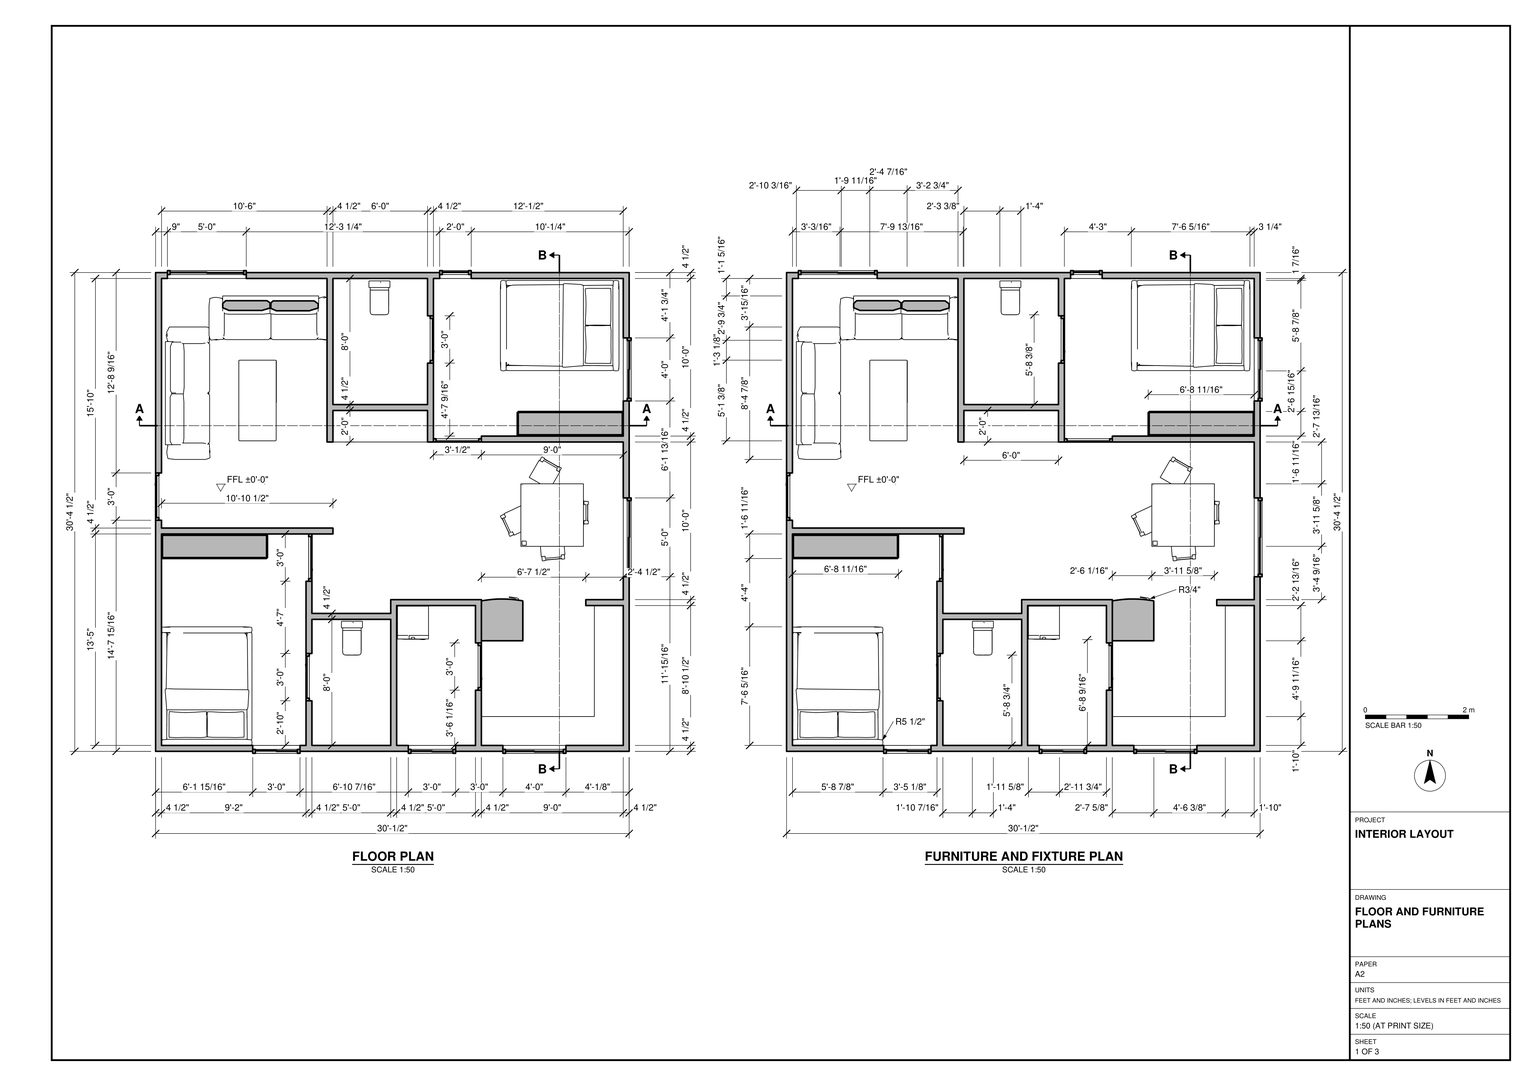
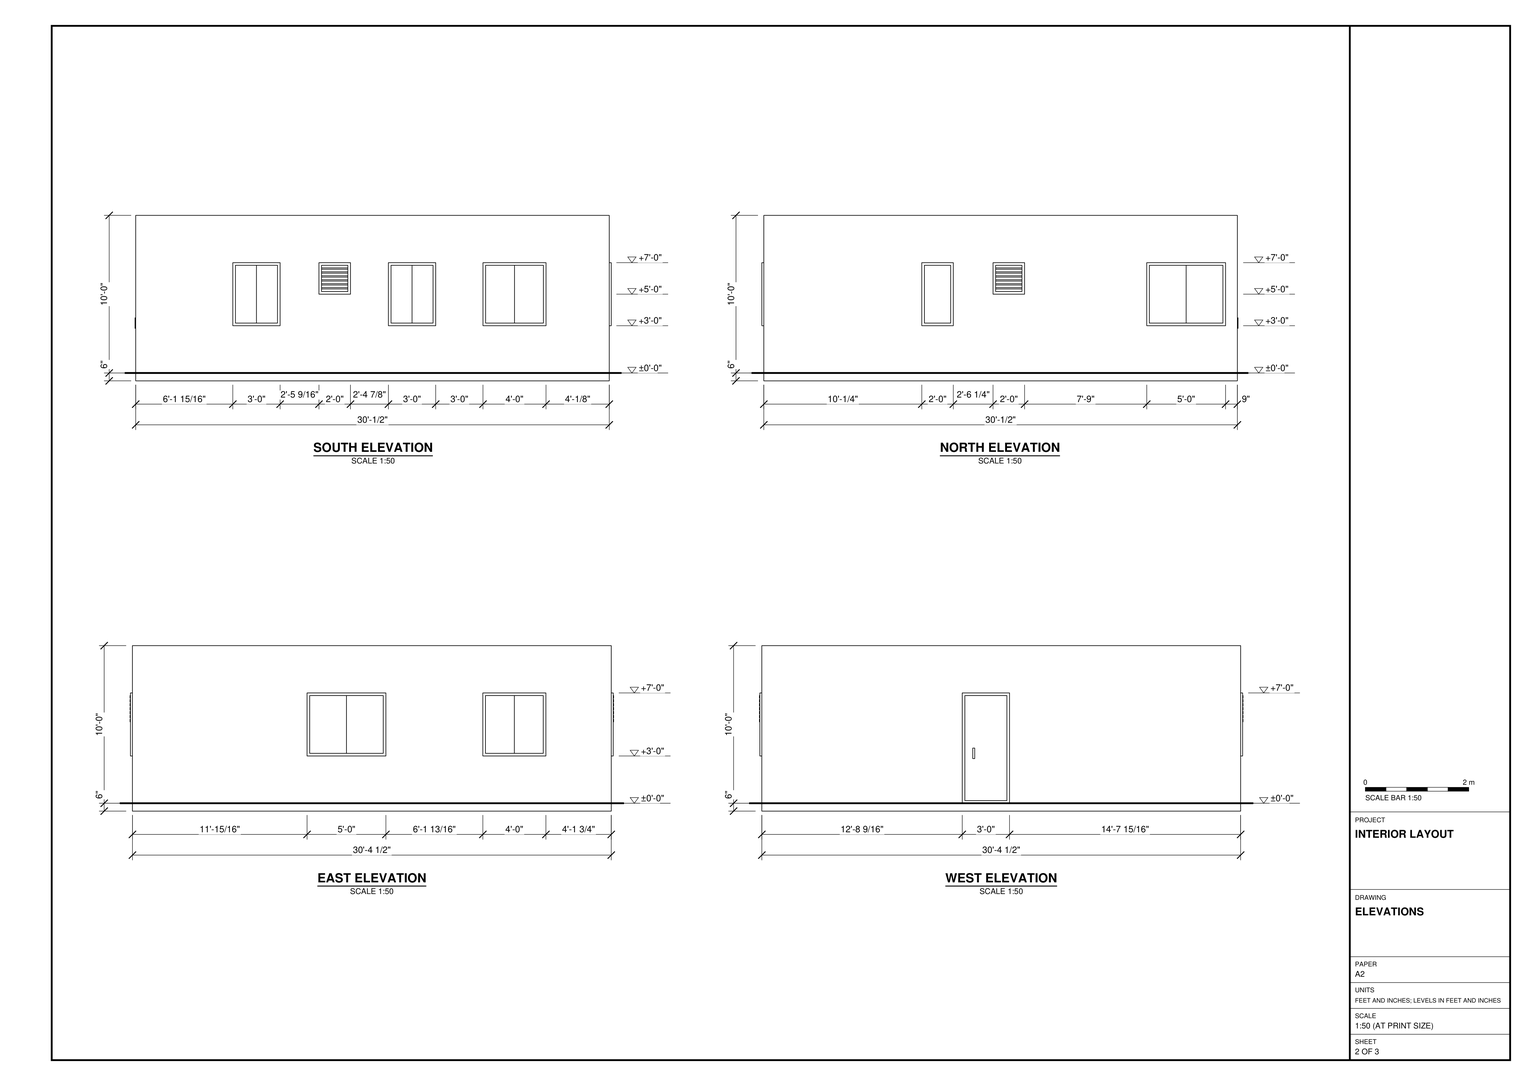
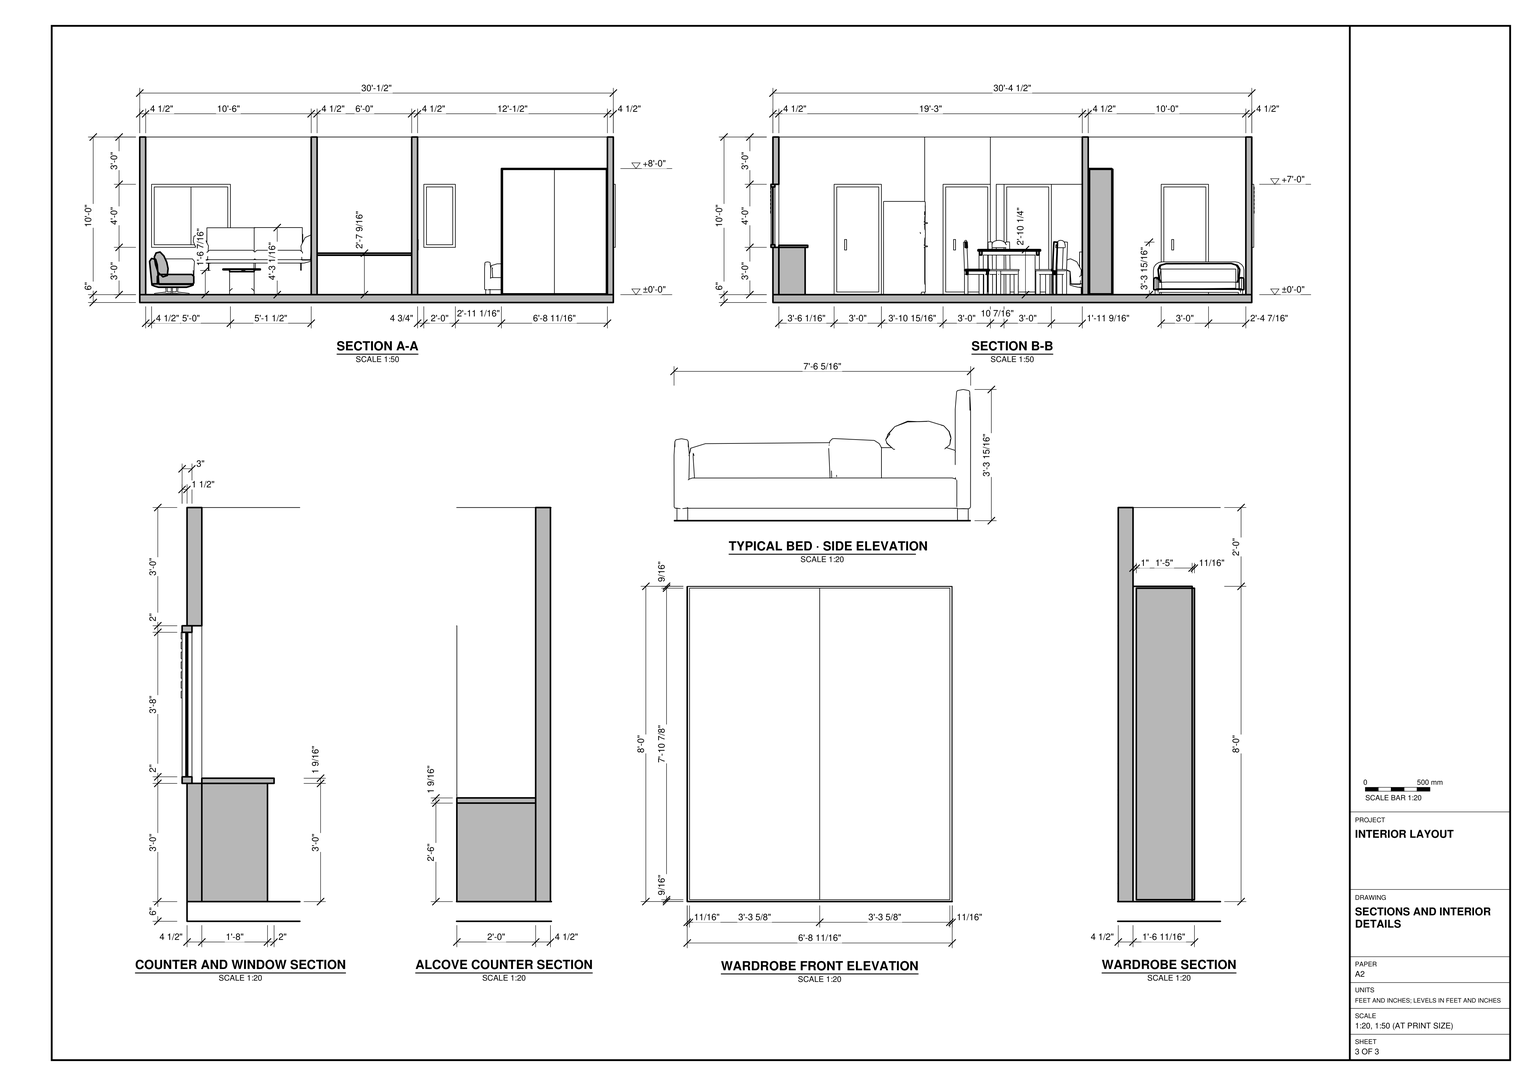
Build the single-storey interior in SketchUp from task_files/diagram_01.pdf. Work in feet and inches. Set the finished floor at ±0'-0" and orient the model with north at the top of the plan. The overall model extents are 30'-2 1/2" east to west, 30'-8 1/8" north to south and 10'-6" high.

Model the 6" floor slab and the 4 1/2" walls. Use the floor plan to set out the partitions and doorways, and the elevations to locate the west entry, framed windows and louvred openings. Keep the living area in the northwest open to the dining area on the east. Place the bedrooms in the northeast and southwest, with the toilet rooms, laundry space and kitchen arranged as shown.

Use the furniture plan to position the seating and low table, dining set, beds, wardrobes, toilet fixtures and appliances. Use the sections and interior details to size the beds and wardrobes and to distinguish the shallow alcove counter from the kitchen counter beneath the window. Decor and loose items, including appliances, may be any suitable library components.

Keep the shell elements and each furniture or joinery piece in separate groups or components, and use components for repeated parts. Save one SketchUp model as output_files/furnished_two_bedroom_interior_and_its_enclosing_shell.skp.

# SketchUp Ruby script. Lengths in inches.
U = 1.inch
M = Sketchup.active_model
def pt(a) = Geom::Point3d.new(a.map { |v| v * U })
def face(e, loops, mat)
  f = e.add_face(loops[0].map { |a| pt(a) })
  loops[1..].each { |l| e.add_face(l.map { |a| pt(a) }).erase! }
  f.material = f.back_material = mat if mat
  f
end
# faces: each face lists its corners as indices into pts; further lists are holes
def faces(e, pts, list, mat = nil) = list.each { |f| face(e, (f[0].is_a?(Array) ? f : [f]).map { |l| l.map { |i| pts[i] } }, mat) }
# xy, xz, yz: faces in a plane at the given z, y or x. An outline is a flat list of corners, or four numbers for a rectangle; further outlines are holes
def ring(l) = l.size == 4 ? [[l[0], l[1]], [l[2], l[1]], [l[2], l[3]], [l[0], l[3]]] : l.each_slice(2).to_a
def flat(e, list, mat, &to3) = list.each { |f| face(e, (f[0].is_a?(Array) ? f : [f]).map { |l| ring(l).map { |u, v| to3.(u, v) } }, mat) }
def xy(e, z, list, mat = nil) = flat(e, list, mat) { |x, y| [x, y, z] }
def xz(e, y, list, mat = nil) = flat(e, list, mat) { |x, z| [x, y, z] }
def yz(e, x, list, mat = nil) = flat(e, list, mat) { |y, z| [x, y, z] }
def lines(e, pts, list) = list.each { |a, b| e.add_line(pt(pts[a]), pt(pts[b])) }
# prism: a flat outline (further loops are holes) pulled along v
def prism(e, loops, v, mat = nil)
  f = face(e, loops, mat); d = Geom::Vector3d.new(v.map { |x| x * U })
  f.pushpull(f.normal.samedirection?(d) ? d.length : -d.length)
end
def box(e, o, s, mat = nil) = prism(e, [[o, [o[0] + s[0], o[1], o[2]], [o[0] + s[0], o[1] + s[1], o[2]], [o[0], o[1] + s[1], o[2]]]], [0, 0, s[2]], mat)
def at(x, y, z, deg = 0) = Geom::Transformation.translation(pt([x, y, z])) * Geom::Transformation.rotation(ORIGIN, Z_AXIS, deg.degrees)
def axes(o, x, y, z) = Geom::Transformation.new([*x, 0, *y, 0, *z, 0, *pt(o).to_a, 1])
def part(name) = M.definitions.add(name)
# library, detail: a bought-in or finely detailed component or shape, given as its bounding box
def library(name, o, s) = part(name).tap { |d| box(d.entities, o, s) }
def detail(e, o, s) = box(e.add_group.entities, o, s)
def put(e, d, t, mat = nil) = e.add_instance(d, t).tap { |i| i.material = mat if mat }
def group(e, t, mat = nil) = e.add_group.tap { |g| g.transformation = t; g.material = mat if mat }.entities
root = M.entities
M.materials.add("Glass Thin Clear 001").color = [0, 0, 0]
M.materials["Glass Thin Clear 001"].alpha = 0.1
M.materials.add("Marble Black 100cm").color = [32, 32, 32]
M.materials.add("Marble White 100cm").color = [222, 222, 222]
M.materials.add("Metal Sandblasted Black 200cm").color = [86, 90, 95]
M.materials.add("Oak Square Panels Rinascimento 240cm").color = [166, 152, 134]
M.materials.add("Porcelain B02 Orange 10cm").color = [208, 126, 69]
M.materials.add("Porcelain Dusk Blue Matte 001").color = [122, 143, 157]
c1 = library("Toilet Bowl 127 010",[-8,-12.9,0],[16,25.8,38.91])
c2 = library("Slow",[-50.42,-21.27,0],[100.85,42.21,32.64])
c3 = library("Toy Table Set 40-09",[-39.37,-33.7,0],[66.93,79.21,41.36])
c4 = library("Table 142 031",[-30.7,-14.21,0],[61.4,28.42,19.53])
c5 = library("Washer 001",[-11.8125,-12.73,0],[23.63,25.47,33.9])
c6 = library("Eva Bed",[-34.4,-44.85,0.04],[68.9,90.3,39.91])
c7 = library("Fridge 143 008",[-15.8,-16.72,0],[31.6,33.44,70.99])
c8 = part("Group\#23")
box(c8.entities,[0,0,0],[20,0.31,2])
c9 = part("Group\#25")
box(c9.entities,[0,-0.31,0],[28,0.31,44])
c10 = part("Group\#27")
box(c10.entities,[0,0,0],[16,0.31,44])
c11 = part("Group\#29")
box(c11.entities,[0,-0.31,0],[20,0.31,2])
c12 = part("Group\#31")
box(c12.entities,[0,0,0],[16,0.31,44])
c13 = part("Group\#33")
box(c13.entities,[0,0,0],[22,0.31,44])
c14 = part("Group\#35")
box(c14.entities,[-0.31,0,0],[0.31,28,44])
c15 = part("Group\#37")
box(c15.entities,[-0.31,0,0],[0.31,22,44])
put(root,c1,at(170.88,347.08,0))
put(root,c1,at(149.95,87.98,0))
put(root,c2,axes([88.06,331.77,18.43],[0.93,0,0],[0,0.8,0],[0,0,1]))
put(root,c3,at(302.34,180.52,0))
put(root,c4,at(78.0625,268.91,0,90))
put(root,c5,at(196.4375,99.61,0))
put(root,c6,at(307.82,325.96,0,-90))
put(root,c6,at(39.5,51.76,-0.04,-180))
put(root,c7,at(264.3,102.72,0,-180))
put(root,c2,axes([24.93,274.45,0],[0,1,0],[-0.81,0,0],[0,0,1]))
g1 = group(root,at(0.5,1.81,0))
xy(g1,0,[[0,0,0,175.9375,4.5,175.9375,4.5,170,135,170,135,165.5,4.5,165.5,4.5,4.5,114.5,4.5,114.5,38.5,119,38.5,119,4.5,179,4.5,179,100.5,119,100.5,119,74.5,114.5,74.5,114.5,129.5,119,129.5,119,105,179,105,179,115.5,248,115.5,248,82.5625,243.5,82.5625,243.5,111,183.5,111,183.5,4.5,243.5,4.5,243.5,46.5625,248,46.5625,248,4.5,356,4.5,356,111,327.5,111,327.5,115.5,356,115.5,356,235.5,248,235.5,248,240,356,240,356,360,211.5,360,211.5,331.5625,207,331.5625,207,360,135,360,135,264,207,264,207,295.5625,211.5,295.5625,211.5,235.5,207,235.5,207,259.5,135,259.5,135,235.5,130.5,235.5,130.5,360,4.5,360,4.5,211.9375,0,211.9375,0,364.5,360.5,364.5,360.5,0]],"Porcelain Dusk Blue Matte 001")
xy(g1,36,[[73.9375,0,109.9375,4.5],[192.375,0,228.375,4.5],[264.375,0,312.375,4.5],[356,132.9375,360.5,192.9375],[356,266.75,360.5,314.75],
  [9,360,69,364.5],[216.25,360,240.25,364.5]],"Porcelain Dusk Blue Matte 001")
xy(g1,60,[[139.5,0,163.5,4.5],[162,360,186,364.5]],"Porcelain Dusk Blue Matte 001")
xy(g1,84,[[73.9375,0,109.9375,4.5],[139.5,0,163.5,4.5],[192.375,0,228.375,4.5],[264.375,0,312.375,4.5],[114.5,38.5,119,74.5],
  [243.5,46.5625,248,82.5625],[114.5,129.5,119,165.5],[356,132.9375,360.5,192.9375],[130.5,170,135,235.5],[0,175.9375,4.5,211.9375],
  [211.5,235.5,248,240],[356,266.75,360.5,314.75],[207,295.5625,211.5,331.5625],[9,360,69,364.5],[162,360,186,364.5],
  [216.25,360,240.25,364.5]],"Porcelain Dusk Blue Matte 001")
xy(g1,120,[[[0,0,360.5,364.5],[248,4.5,248,115.5,179,115.5,179,105,119,105,119,165.5,135,165.5,135,259.5,207,259.5,207,235.5,356,235.5,356,115.5,327.5,115.5,327.5,111,356,111,356,4.5],[4.5,170,130.5,360],[4.5,4.5,114.5,165.5],[211.5,240,356,360],[135,264,207,360],[183.5,4.5,243.5,111],[119,4.5,179,100.5]]],"Porcelain Dusk Blue Matte 001")
xz(g1,0,[[[0,0,360.5,120],[264.375,36,312.375,84],[73.9375,36,109.9375,84],[192.375,36,228.375,84],[139.5,60,163.5,84]]],"Porcelain Dusk Blue Matte 001")
xz(g1,4.5,[[[4.5,0,114.5,120],[73.9375,36,109.9375,84]],[[119,0,179,120],[139.5,60,163.5,84]],[[183.5,0,243.5,120],[192.375,36,228.375,84]],[[248,0,356,120],[264.375,36,312.375,84]]],"Porcelain Dusk Blue Matte 001")
xz(g1,38.5,[[114.5,0,119,84]],"Porcelain Dusk Blue Matte 001")
xz(g1,46.5625,[[243.5,0,248,84]],"Porcelain Dusk Blue Matte 001")
xz(g1,74.5,[[114.5,0,119,84]],"Porcelain Dusk Blue Matte 001")
xz(g1,82.5625,[[243.5,0,248,84]],"Porcelain Dusk Blue Matte 001")
xz(g1,100.5,[[119,0,179,120]],"Porcelain Dusk Blue Matte 001")
xz(g1,105,[[119,0,179,120]],"Porcelain Dusk Blue Matte 001")
xz(g1,111,[[183.5,0,243.5,120],[327.5,0,356,120]],"Porcelain Dusk Blue Matte 001")
xz(g1,115.5,[[179,0,248,120],[327.5,0,356,120]],"Porcelain Dusk Blue Matte 001")
xz(g1,129.5,[[114.5,0,119,84]],"Porcelain Dusk Blue Matte 001")
xz(g1,132.9375,[[356,36,360.5,84]],"Porcelain Dusk Blue Matte 001")
xz(g1,165.5,[[4.5,0,135,0,135,120,119,120,119,84,114.5,84,114.5,120,4.5,120]],"Porcelain Dusk Blue Matte 001")
xz(g1,170,[[4.5,0,4.5,120,130.5,120,130.5,84,135,84,135,0]],"Porcelain Dusk Blue Matte 001")
xz(g1,175.9375,[[0,0,4.5,84]],"Porcelain Dusk Blue Matte 001")
xz(g1,192.9375,[[356,36,360.5,84]],"Porcelain Dusk Blue Matte 001")
xz(g1,211.9375,[[0,0,4.5,84]],"Porcelain Dusk Blue Matte 001")
xz(g1,235.5,[[130.5,0,135,84],[207,0,211.5,0,211.5,84,248,84,248,0,356,0,356,120,207,120]],"Porcelain Dusk Blue Matte 001")
xz(g1,240,[[248,0,248,84,211.5,84,211.5,120,356,120,356,0]],"Porcelain Dusk Blue Matte 001")
xz(g1,259.5,[[135,0,207,120]],"Porcelain Dusk Blue Matte 001")
xz(g1,264,[[135,0,207,120]],"Porcelain Dusk Blue Matte 001")
xz(g1,266.75,[[356,36,360.5,84]],"Porcelain Dusk Blue Matte 001")
xz(g1,295.5625,[[207,0,211.5,84]],"Porcelain Dusk Blue Matte 001")
xz(g1,314.75,[[356,36,360.5,84]],"Porcelain Dusk Blue Matte 001")
xz(g1,331.5625,[[207,0,211.5,84]],"Porcelain Dusk Blue Matte 001")
xz(g1,360,[[[4.5,0,130.5,120],[9,36,69,84]],[[135,0,207,120],[162,60,186,84]],[[211.5,0,356,120],[216.25,36,240.25,84]]],"Porcelain Dusk Blue Matte 001")
xz(g1,364.5,[[[0,0,360.5,120],[9,36,69,84],[216.25,36,240.25,84],[162,60,186,84]]],"Porcelain Dusk Blue Matte 001")
yz(g1,0,[[0,0,0,120,364.5,120,364.5,0,211.9375,0,211.9375,84,175.9375,84,175.9375,0]],"Porcelain Dusk Blue Matte 001")
yz(g1,4.5,[[4.5,0,165.5,120],[170,0,175.9375,0,175.9375,84,211.9375,84,211.9375,0,360,0,360,120,170,120]],"Porcelain Dusk Blue Matte 001")
yz(g1,9,[[360,36,364.5,84]],"Porcelain Dusk Blue Matte 001")
yz(g1,69,[[360,36,364.5,84]],"Porcelain Dusk Blue Matte 001")
yz(g1,73.9375,[[0,36,4.5,84]],"Porcelain Dusk Blue Matte 001")
yz(g1,109.9375,[[0,36,4.5,84]],"Porcelain Dusk Blue Matte 001")
yz(g1,114.5,[[4.5,0,4.5,120,165.5,120,165.5,84,129.5,84,129.5,0,74.5,0,74.5,84,38.5,84,38.5,0]],"Porcelain Dusk Blue Matte 001")
yz(g1,119,[[4.5,0,38.5,0,38.5,84,74.5,84,74.5,0,100.5,0,100.5,120,4.5,120],[105,0,129.5,0,129.5,84,165.5,84,165.5,120,105,120]],"Porcelain Dusk Blue Matte 001")
yz(g1,130.5,[[235.5,0,235.5,84,170,84,170,120,360,120,360,0]],"Porcelain Dusk Blue Matte 001")
yz(g1,135,[[165.5,0,170,0,170,84,235.5,84,235.5,0,259.5,0,259.5,120,165.5,120],[264,0,360,120]],"Porcelain Dusk Blue Matte 001")
yz(g1,139.5,[[0,60,4.5,84]],"Porcelain Dusk Blue Matte 001")
yz(g1,162,[[360,60,364.5,84]],"Porcelain Dusk Blue Matte 001")
yz(g1,163.5,[[0,60,4.5,84]],"Porcelain Dusk Blue Matte 001")
yz(g1,179,[[4.5,0,100.5,120],[105,0,115.5,120]],"Porcelain Dusk Blue Matte 001")
yz(g1,183.5,[[4.5,0,111,120]],"Porcelain Dusk Blue Matte 001")
yz(g1,186,[[360,60,364.5,84]],"Porcelain Dusk Blue Matte 001")
yz(g1,192.375,[[0,36,4.5,84]],"Porcelain Dusk Blue Matte 001")
yz(g1,207,[[235.5,0,259.5,120],[264,0,264,120,360,120,360,0,331.5625,0,331.5625,84,295.5625,84,295.5625,0]],"Porcelain Dusk Blue Matte 001")
yz(g1,211.5,[[235.5,0,295.5625,0,295.5625,84,331.5625,84,331.5625,0,360,0,360,120,240,120,240,84,235.5,84]],"Porcelain Dusk Blue Matte 001")
yz(g1,216.25,[[360,36,364.5,84]],"Porcelain Dusk Blue Matte 001")
yz(g1,228.375,[[0,36,4.5,84]],"Porcelain Dusk Blue Matte 001")
yz(g1,240.25,[[360,36,364.5,84]],"Porcelain Dusk Blue Matte 001")
yz(g1,243.5,[[4.5,0,4.5,120,111,120,111,0,82.5625,0,82.5625,84,46.5625,84,46.5625,0]],"Porcelain Dusk Blue Matte 001")
yz(g1,248,[[4.5,0,46.5625,0,46.5625,84,82.5625,84,82.5625,0,115.5,0,115.5,120,4.5,120],[235.5,0,240,84]],"Porcelain Dusk Blue Matte 001")
yz(g1,264.375,[[0,36,4.5,84]],"Porcelain Dusk Blue Matte 001")
yz(g1,312.375,[[0,36,4.5,84]],"Porcelain Dusk Blue Matte 001")
yz(g1,327.5,[[111,0,115.5,120]],"Porcelain Dusk Blue Matte 001")
yz(g1,356,[[4.5,0,111,120],[[115.5,0,235.5,120],[132.9375,36,192.9375,84]],[[240,0,360,120],[266.75,36,314.75,84]]],"Porcelain Dusk Blue Matte 001")
yz(g1,360.5,[[[0,0,364.5,120],[132.9375,36,192.9375,84],[266.75,36,314.75,84]]],"Porcelain Dusk Blue Matte 001")
p = [[114.5,74.5,0],[114.5,38.5,0],[248,46.5625,0],[248,82.5625,0],[211.5,235.5,0],[248,235.5,0]]
lines(g1,p,[[0,1],[2,3],[4,5]])
g2 = group(g1,at(114.5,38.5,0))
prism(g2,[[[0,0,0],[0,0,84],[0,36,84],[0,36,0]],[[0,2,2],[0,34,2],[0,34,82],[0,2,82]]],[2.5,0,0],"Metal Sandblasted Black 200cm")
g3 = group(g2,at(0,2,2))
box(g3,[0,0,0],[0.71,32,80],"Oak Square Panels Rinascimento 240cm")
g4 = group(g3,at(0,26,32),"Metal Sandblasted Black 200cm")
box(g4,[-0.5,-1.5,0],[0.5,1.5,8])
g5 = group(g1,at(248,46.5625,0))
prism(g5,[[[0,36,0],[0,36,84],[0,0,84],[0,0,0]],[[0,34,2],[0,2,2],[0,2,82],[0,34,82]]],[-2.5,0,0],"Metal Sandblasted Black 200cm")
g6 = group(g5,at(0,2,2))
box(g6,[-0.71,0,0],[0.71,32,80],"Oak Square Panels Rinascimento 240cm")
g7 = group(g6,at(0,6,32),"Metal Sandblasted Black 200cm")
box(g7,[0,0,0],[0.5,1.5,8])
g8 = group(g1,at(211.5,235.5,0))
prism(g8,[[[36.5,0,0],[36.5,0,84],[0,0,84],[0,0,0]],[[34.5,0,82],[34.5,0,2],[2,0,2],[2,0,82]]],[0,2.5,0],"Metal Sandblasted Black 200cm")
g9 = group(g8,at(2,0,2))
box(g9,[0,0,0],[32.5,0.71,80],"Oak Square Panels Rinascimento 240cm")
g10 = group(g9,at(6,0,32))
box(g10,[0,-0.1875,0],[1.5,0.1875,8],"Metal Sandblasted Black 200cm")
g11 = group(g1,at(216.25,364.5,36))
prism(g11,[[[0,1.5,0],[0,1.5,48],[24,1.5,48],[24,1.5,0]],[[22,1.5,2],[22,1.5,46],[2,1.5,46],[2,1.5,2]]],[0,-3,0],"Metal Sandblasted Black 200cm")
g12 = group(g11,at(2,0.5,2))
box(g12,[0,-0.31,0],[20,0.31,44],"Glass Thin Clear 001")
g13 = group(g1,at(162,364.5,60))
xy(g13,0,[[0,-1.5,24,1.5]],"Metal Sandblasted Black 200cm")
xy(g13,2,[[2,-1.5,22,1.5]],"Metal Sandblasted Black 200cm")
xy(g13,22,[[2,-1.5,22,1.5]],"Metal Sandblasted Black 200cm")
xy(g13,24,[[0,-1.5,24,1.5]],"Metal Sandblasted Black 200cm")
xz(g13,-1.5,[[[0,0,24,24],[2,2,22,22]]],"Metal Sandblasted Black 200cm")
xz(g13,1.5,[[[0,0,24,24],[2,2,22,22]]],"Metal Sandblasted Black 200cm")
yz(g13,0,[[-1.5,0,1.5,24]],"Metal Sandblasted Black 200cm")
yz(g13,2,[[-1.5,2,1.5,22]],"Metal Sandblasted Black 200cm")
yz(g13,22,[[-1.5,2,1.5,22]],"Metal Sandblasted Black 200cm")
yz(g13,24,[[-1.5,0,1.5,24]],"Metal Sandblasted Black 200cm")
put(g13,c8,at(2,1.5,20),"Glass Thin Clear 001")
put(g13,c8,at(2,1.5,17),"Glass Thin Clear 001")
put(g13,c8,at(2,1.5,14),"Glass Thin Clear 001")
put(g13,c8,at(2,1.5,11),"Glass Thin Clear 001")
put(g13,c8,at(2,1.5,8),"Glass Thin Clear 001")
put(g13,c8,at(2,1.5,5),"Glass Thin Clear 001")
put(g13,c8,at(2,1.5,2),"Glass Thin Clear 001")
g14 = group(g1,at(9,364.5,36))
xy(g14,0,[[0,-1.5,60,1.5]],"Metal Sandblasted Black 200cm")
xy(g14,2,[[2,-1.5,58,1.5]],"Metal Sandblasted Black 200cm")
xy(g14,46,[[2,-1.5,58,1.5]],"Metal Sandblasted Black 200cm")
xy(g14,48,[[0,-1.5,60,1.5]],"Metal Sandblasted Black 200cm")
xz(g14,-1.5,[[[0,0,60,48],[2,2,58,46]]],"Metal Sandblasted Black 200cm")
xz(g14,1.5,[[[0,0,60,48],[2,2,58,46]]],"Metal Sandblasted Black 200cm")
yz(g14,0,[[-1.5,0,1.5,48]],"Metal Sandblasted Black 200cm")
yz(g14,2,[[-1.5,2,1.5,46]],"Metal Sandblasted Black 200cm")
yz(g14,58,[[-1.5,2,1.5,46]],"Metal Sandblasted Black 200cm")
yz(g14,60,[[-1.5,0,1.5,48]],"Metal Sandblasted Black 200cm")
put(g14,c9,at(30,-0.0625,2),"Glass Thin Clear 001")
put(g14,c9,at(2,0.25,2),"Glass Thin Clear 001")
g15 = group(g1,at(73.9375,0,36))
xy(g15,0,[[0,-1.5,36,1.5]],"Metal Sandblasted Black 200cm")
xy(g15,2,[[2,-1.5,34,1.5]],"Metal Sandblasted Black 200cm")
xy(g15,46,[[2,-1.5,34,1.5]],"Metal Sandblasted Black 200cm")
xy(g15,48,[[0,-1.5,36,1.5]],"Metal Sandblasted Black 200cm")
xz(g15,-1.5,[[[0,0,36,48],[2,2,34,46]]],"Metal Sandblasted Black 200cm")
xz(g15,1.5,[[[0,0,36,48],[2,2,34,46]]],"Metal Sandblasted Black 200cm")
yz(g15,0,[[-1.5,0,1.5,48]],"Metal Sandblasted Black 200cm")
yz(g15,2,[[-1.5,2,1.5,46]],"Metal Sandblasted Black 200cm")
yz(g15,34,[[-1.5,2,1.5,46]],"Metal Sandblasted Black 200cm")
yz(g15,36,[[-1.5,0,1.5,48]],"Metal Sandblasted Black 200cm")
put(g15,c10,at(2,0.375,2),"Glass Thin Clear 001")
put(g15,c10,at(18,0.06,2),"Glass Thin Clear 001")
g16 = group(g1,at(139.5,0,60))
xy(g16,0,[[0,-1.5,24,1.5]],"Metal Sandblasted Black 200cm")
xy(g16,2,[[2,-1.5,22,1.5]],"Metal Sandblasted Black 200cm")
xy(g16,22,[[2,-1.5,22,1.5]],"Metal Sandblasted Black 200cm")
xy(g16,24,[[0,-1.5,24,1.5]],"Metal Sandblasted Black 200cm")
xz(g16,-1.5,[[[0,0,24,24],[2,2,22,22]]],"Metal Sandblasted Black 200cm")
xz(g16,1.5,[[[0,0,24,24],[2,2,22,22]]],"Metal Sandblasted Black 200cm")
yz(g16,0,[[-1.5,0,1.5,24]],"Metal Sandblasted Black 200cm")
yz(g16,2,[[-1.5,2,1.5,22]],"Metal Sandblasted Black 200cm")
yz(g16,22,[[-1.5,2,1.5,22]],"Metal Sandblasted Black 200cm")
yz(g16,24,[[-1.5,0,1.5,24]],"Metal Sandblasted Black 200cm")
put(g16,c11,at(2,-1.5,20),"Glass Thin Clear 001")
put(g16,c11,at(2,-1.5,17),"Glass Thin Clear 001")
put(g16,c11,at(2,-1.5,14),"Glass Thin Clear 001")
put(g16,c11,at(2,-1.5,11),"Glass Thin Clear 001")
put(g16,c11,at(2,-1.5,8),"Glass Thin Clear 001")
put(g16,c11,at(2,-1.5,5),"Glass Thin Clear 001")
put(g16,c11,at(2,-1.5,2),"Glass Thin Clear 001")
g17 = group(g1,at(192.375,0,36))
xy(g17,0,[[0,-1.5,36,1.5]],"Metal Sandblasted Black 200cm")
xy(g17,2,[[2,-1.5,34,1.5]],"Metal Sandblasted Black 200cm")
xy(g17,46,[[2,-1.5,34,1.5]],"Metal Sandblasted Black 200cm")
xy(g17,48,[[0,-1.5,36,1.5]],"Metal Sandblasted Black 200cm")
xz(g17,-1.5,[[[0,0,36,48],[2,2,34,46]]],"Metal Sandblasted Black 200cm")
xz(g17,1.5,[[[0,0,36,48],[2,2,34,46]]],"Metal Sandblasted Black 200cm")
yz(g17,0,[[-1.5,0,1.5,48]],"Metal Sandblasted Black 200cm")
yz(g17,2,[[-1.5,2,1.5,46]],"Metal Sandblasted Black 200cm")
yz(g17,34,[[-1.5,2,1.5,46]],"Metal Sandblasted Black 200cm")
yz(g17,36,[[-1.5,0,1.5,48]],"Metal Sandblasted Black 200cm")
put(g17,c12,at(2,0.0625,2),"Glass Thin Clear 001")
put(g17,c12,at(18,-0.25,2),"Glass Thin Clear 001")
g18 = group(g1,at(264.375,0,36))
xy(g18,0,[[0,-1.5,48,1.5]],"Metal Sandblasted Black 200cm")
xy(g18,2,[[2,-1.5,46,1.5]],"Metal Sandblasted Black 200cm")
xy(g18,46,[[2,-1.5,46,1.5]],"Metal Sandblasted Black 200cm")
xy(g18,48,[[0,-1.5,48,1.5]],"Metal Sandblasted Black 200cm")
xz(g18,-1.5,[[[0,0,48,48],[2,2,46,46]]],"Metal Sandblasted Black 200cm")
xz(g18,1.5,[[[0,0,48,48],[2,2,46,46]]],"Metal Sandblasted Black 200cm")
yz(g18,0,[[-1.5,0,1.5,48]],"Metal Sandblasted Black 200cm")
yz(g18,2,[[-1.5,2,1.5,46]],"Metal Sandblasted Black 200cm")
yz(g18,46,[[-1.5,2,1.5,46]],"Metal Sandblasted Black 200cm")
yz(g18,48,[[-1.5,0,1.5,48]],"Metal Sandblasted Black 200cm")
put(g18,c13,at(2,0,2),"Glass Thin Clear 001")
put(g18,c13,at(24,-0.31,2),"Glass Thin Clear 001")
g19 = group(g1,at(360.5,132.9375,36))
xy(g19,0,[[-1.5,0,1.5,60]],"Metal Sandblasted Black 200cm")
xy(g19,2,[[-1.5,2,1.5,58]],"Metal Sandblasted Black 200cm")
xy(g19,46,[[-1.5,2,1.5,58]],"Metal Sandblasted Black 200cm")
xy(g19,48,[[-1.5,0,1.5,60]],"Metal Sandblasted Black 200cm")
xz(g19,0,[[-1.5,0,1.5,48]],"Metal Sandblasted Black 200cm")
xz(g19,2,[[-1.5,2,1.5,46]],"Metal Sandblasted Black 200cm")
xz(g19,58,[[-1.5,2,1.5,46]],"Metal Sandblasted Black 200cm")
xz(g19,60,[[-1.5,0,1.5,48]],"Metal Sandblasted Black 200cm")
yz(g19,-1.5,[[[0,0,60,48],[2,2,58,46]]],"Metal Sandblasted Black 200cm")
yz(g19,1.5,[[[0,0,60,48],[2,2,58,46]]],"Metal Sandblasted Black 200cm")
put(g19,c14,at(-0.0625,2,2),"Glass Thin Clear 001")
put(g19,c14,at(0.25,30,2),"Glass Thin Clear 001")
g20 = group(g1,at(360.5,266.75,36))
xy(g20,0,[[-1.5,0,1.5,48]],"Metal Sandblasted Black 200cm")
xy(g20,2,[[-1.5,2,1.5,46]],"Metal Sandblasted Black 200cm")
xy(g20,46,[[-1.5,2,1.5,46]],"Metal Sandblasted Black 200cm")
xy(g20,48,[[-1.5,0,1.5,48]],"Metal Sandblasted Black 200cm")
xz(g20,0,[[-1.5,0,1.5,48]],"Metal Sandblasted Black 200cm")
xz(g20,2,[[-1.5,2,1.5,46]],"Metal Sandblasted Black 200cm")
xz(g20,46,[[-1.5,2,1.5,46]],"Metal Sandblasted Black 200cm")
xz(g20,48,[[-1.5,0,1.5,48]],"Metal Sandblasted Black 200cm")
yz(g20,-1.5,[[[0,0,48,48],[2,2,46,46]]],"Metal Sandblasted Black 200cm")
yz(g20,1.5,[[[0,0,48,48],[2,2,46,46]]],"Metal Sandblasted Black 200cm")
put(g20,c15,at(-0.125,2,2),"Glass Thin Clear 001")
put(g20,c15,at(0.19,24,2),"Glass Thin Clear 001")
g21 = group(root,at(0.5,177.75,0))
prism(g21,[[[0,36,0],[0,0,0],[0,0,84],[0,36,84]],[[0,2,82],[0,2,2],[0,34,2],[0,34,82]]],[2.5,0,0],"Metal Sandblasted Black 200cm")
g22 = group(g21,at(0,2,2))
box(g22,[0,0,0],[0.71,32,80],"Oak Square Panels Rinascimento 240cm")
g23 = group(g22,at(0,26,32),"Metal Sandblasted Black 200cm")
box(g23,[-0.5,-1.5,0],[0.5,1.5,8])
g24 = group(root,at(119.5,131.31,0))
prism(g24,[[[0,36,0],[0,36,84],[0,0,84],[0,0,0]],[[0,34,82],[0,34,2],[0,2,2],[0,2,82]]],[-2.5,0,0],"Metal Sandblasted Black 200cm")
g25 = group(g24,at(0,2,2))
box(g25,[-0.71,0,0],[0.71,32,80],"Oak Square Panels Rinascimento 240cm")
g26 = group(g25,at(0,6,32),"Metal Sandblasted Black 200cm")
box(g26,[0,0,0],[0.5,1.5,8])
g27 = group(root,at(212,297.38,0))
prism(g27,[[[0,0,0],[0,36,0],[0,36,84],[0,0,84]],[[0,34,82],[0,34,2],[0,2,2],[0,2,82]]],[-2.5,0,0],"Metal Sandblasted Black 200cm")
g28 = group(g27,at(0,2,2))
box(g28,[-0.71,0,0],[0.71,32,80],"Oak Square Panels Rinascimento 240cm")
g29 = group(g28,at(0,6,32),"Metal Sandblasted Black 200cm")
box(g29,[0,0,0],[0.5,1.5,8])
g30 = group(root,at(0.5,1.81,0))
box(g30,[0,0,-6],[360.5,364.5,6],"Marble Black 100cm")
g31 = group(root,at(248.5,6.31,0),"Porcelain B02 Orange 10cm")
prism(g31,[[[0,20,0],[88,20,0],[88,106.5,0],[108,106.5,0],[108,0,0],[0,0,0]]],[0,0,36],"Porcelain B02 Orange 10cm")
g32 = group(root,at(336.7,6.31,36),"Marble White 100cm")
prism(g32,[[[19.8,0,0],[-88.2,0,0],[-88.2,22,0],[-2.2,22,0],[-2.2,106.5,0],[19.8,106.5,0]]],[0,0,1.57],"Marble White 100cm")
g33 = group(root,at(135.5,237.31,0),"Porcelain B02 Orange 10cm")
box(g33,[0,0,0],[72,24,30],"Porcelain B02 Orange 10cm")
g34 = group(root,at(135.5,237.31,30),"Marble White 100cm")
box(g34,[0,0,0],[72,24,1.57],"Marble White 100cm")
g35 = group(root,at(275.82,241.81,0),"Porcelain B02 Orange 10cm")
xy(g35,0,[[0,0,80.68,18]],"Porcelain B02 Orange 10cm")
xy(g35,0.57,[[0.71,1,79.97,18]],"Porcelain B02 Orange 10cm")
xy(g35,95.43,[[0.71,1,79.97,18]],"Porcelain B02 Orange 10cm")
xy(g35,96,[[0,0,80.68,18]],"Porcelain B02 Orange 10cm")
xz(g35,0,[[0,0,80.68,96]],"Porcelain B02 Orange 10cm")
xz(g35,1,[[0.71,0.57,79.97,95.43]],"Porcelain B02 Orange 10cm")
xz(g35,18,[[[0.1,0.08,80.58,95.92],[0.71,0.57,79.97,95.43]]],"Porcelain B02 Orange 10cm")
yz(g35,0,[[0,0,18,96]],"Porcelain B02 Orange 10cm")
yz(g35,0.71,[[1,0.57,18,95.43]],"Porcelain B02 Orange 10cm")
yz(g35,79.97,[[1,0.57,18,95.43]],"Porcelain B02 Orange 10cm")
yz(g35,80.68,[[0,0,18,96]],"Porcelain B02 Orange 10cm")
p = [[40.34,18,95.43],[40.34,18,0.57]]
lines(g35,p,[[0,1]])
g36 = group(g35,at(40.34,18,0.57))
box(g36,[0,0,0],[39.63,0.71,94.87],"Porcelain B02 Orange 10cm")
g37 = group(g35,at(0.71,18,0.57))
box(g37,[0,0,0],[39.63,0.71,94.87],"Porcelain B02 Orange 10cm")
g38 = group(root,at(85.68,167.31,0),"Porcelain B02 Orange 10cm")
xy(g38,0,[[-80.68,-18,0,0]],"Porcelain B02 Orange 10cm")
xy(g38,0.57,[[-79.97,-18,-0.71,-1]],"Porcelain B02 Orange 10cm")
xy(g38,95.43,[[-79.97,-18,-0.71,-1]],"Porcelain B02 Orange 10cm")
xy(g38,96,[[-80.68,-18,0,0]],"Porcelain B02 Orange 10cm")
xz(g38,-18,[[[-80.58,0.08,-0.1,95.92],[-79.97,0.57,-0.71,95.43]]],"Porcelain B02 Orange 10cm")
xz(g38,-1,[[-79.97,0.57,-0.71,95.43]],"Porcelain B02 Orange 10cm")
xz(g38,0,[[-80.68,0,0,96]],"Porcelain B02 Orange 10cm")
yz(g38,-80.68,[[-18,0,0,96]],"Porcelain B02 Orange 10cm")
yz(g38,-79.97,[[-18,0.57,-1,95.43]],"Porcelain B02 Orange 10cm")
yz(g38,-0.71,[[-18,0.57,-1,95.43]],"Porcelain B02 Orange 10cm")
yz(g38,0,[[-18,0,0,96]],"Porcelain B02 Orange 10cm")
p = [[-40.34,-18,95.43],[-40.34,-18,0.57]]
lines(g38,p,[[0,1]])
g39 = group(g38,at(-40.34,-18,0.57))
box(g39,[-39.63,-0.71,0],[39.63,0.71,94.87],"Porcelain B02 Orange 10cm")
g40 = group(g38,at(-0.71,-18,0.57))
box(g40,[-39.63,-0.71,0],[39.63,0.71,94.87],"Porcelain B02 Orange 10cm")
